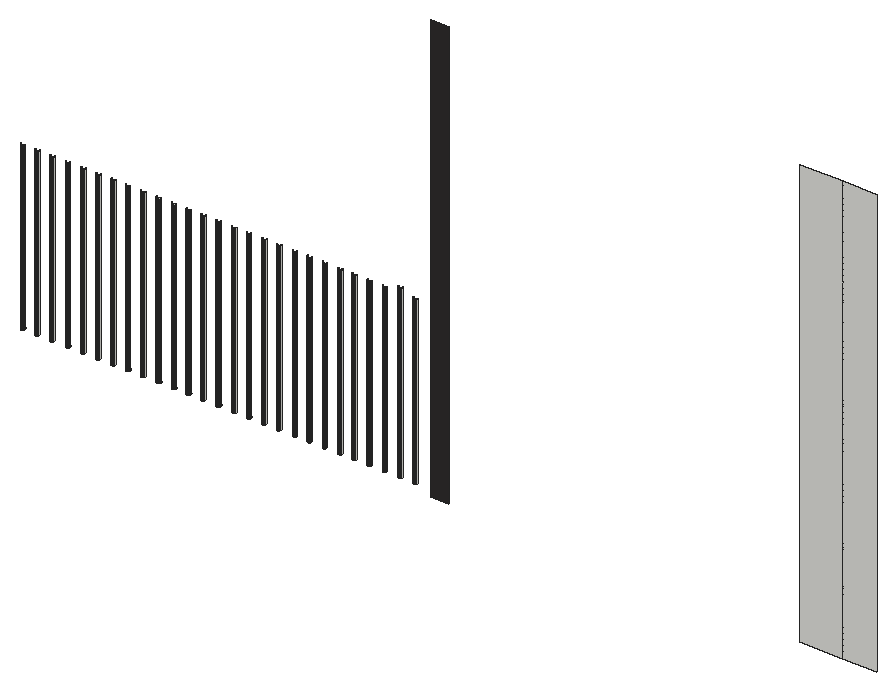
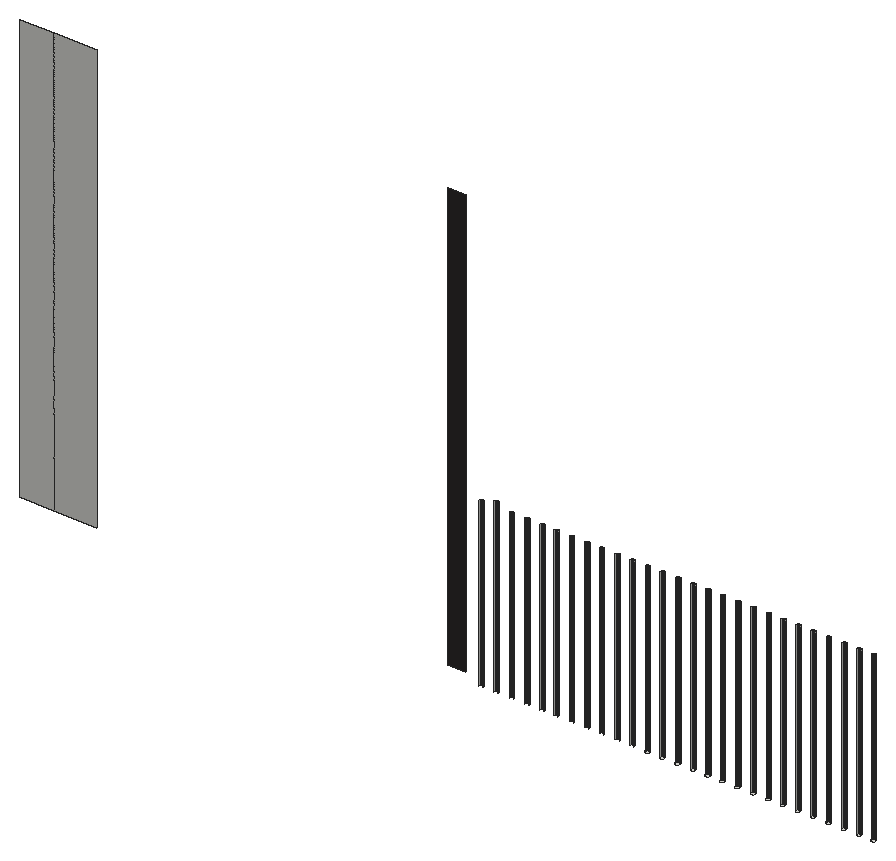
# SketchUp Ruby script. Lengths in inches.
U = 1.inch
M = Sketchup.active_model
def pt(a) = Geom::Point3d.new(a.map { |v| v * U })
def face(e, loops, mat)
  f = e.add_face(loops[0].map { |a| pt(a) })
  loops[1..].each { |l| e.add_face(l.map { |a| pt(a) }).erase! }
  f.material = f.back_material = mat if mat
  f
end
# faces: each face lists its corners as indices into pts; further lists are holes
def faces(e, pts, list, mat = nil) = list.each { |f| face(e, (f[0].is_a?(Array) ? f : [f]).map { |l| l.map { |i| pts[i] } }, mat) }
# xy, xz, yz: faces in a plane at the given z, y or x. An outline is a flat list of corners, or four numbers for a rectangle; further outlines are holes
def ring(l) = l.size == 4 ? [[l[0], l[1]], [l[2], l[1]], [l[2], l[3]], [l[0], l[3]]] : l.each_slice(2).to_a
def flat(e, list, mat, &to3) = list.each { |f| face(e, (f[0].is_a?(Array) ? f : [f]).map { |l| ring(l).map { |u, v| to3.(u, v) } }, mat) }
def xy(e, z, list, mat = nil) = flat(e, list, mat) { |x, y| [x, y, z] }
def xz(e, y, list, mat = nil) = flat(e, list, mat) { |x, z| [x, y, z] }
def yz(e, x, list, mat = nil) = flat(e, list, mat) { |y, z| [x, y, z] }
def lines(e, pts, list) = list.each { |a, b| e.add_line(pt(pts[a]), pt(pts[b])) }
# prism: a flat outline (further loops are holes) pulled along v
def prism(e, loops, v, mat = nil)
  f = face(e, loops, mat); d = Geom::Vector3d.new(v.map { |x| x * U })
  f.pushpull(f.normal.samedirection?(d) ? d.length : -d.length)
end
def box(e, o, s, mat = nil) = prism(e, [[o, [o[0] + s[0], o[1], o[2]], [o[0] + s[0], o[1] + s[1], o[2]], [o[0], o[1] + s[1], o[2]]]], [0, 0, s[2]], mat)
def at(x, y, z, deg = 0) = Geom::Transformation.translation(pt([x, y, z])) * Geom::Transformation.rotation(ORIGIN, Z_AXIS, deg.degrees)
def axes(o, x, y, z) = Geom::Transformation.new([*x, 0, *y, 0, *z, 0, *pt(o).to_a, 1])
def part(name) = M.definitions.add(name)
# library, detail: a bought-in or finely detailed component or shape, given as its bounding box
def library(name, o, s) = part(name).tap { |d| box(d.entities, o, s) }
def detail(e, o, s) = box(e.add_group.entities, o, s)
def put(e, d, t, mat = nil) = e.add_instance(d, t).tap { |i| i.material = mat if mat }
def group(e, t, mat = nil) = e.add_group.tap { |g| g.transformation = t; g.material = mat if mat }.entities
root = M.entities
M.materials.add("Generic\#4").color = [48, 45, 45]
xy(root,819.75,[[365.01,127.81,364.8,127.83,364.6,127.91,364.4375,128.04,364.31,128.21,364.23,128.41,364.2,128.62,364.23,128.83,364.31,129.02,364.4375,129.19,364.6,129.32,364.8,129.4,365.01,129.43,365.22,129.4,365.42,129.32,365.59,129.19,365.71,129.02,365.8,128.83,365.82,128.62,365.8,128.41,365.71,128.21,365.59,128.04,365.42,127.91,365.22,127.83],[370.76,127.81,370.55,127.83,370.35,127.91,370.1875,128.04,370.06,128.21,369.98,128.41,369.95,128.62,369.98,128.83,370.06,129.02,370.1875,129.19,370.35,129.32,370.55,129.4,370.76,129.43,370.97,129.4,371.17,129.32,371.34,129.19,371.46,129.02,371.55,128.83,371.57,128.62,371.55,128.41,371.46,128.21,371.34,128.04,371.17,127.91,370.97,127.83],[376.7,127.81,376.49,127.83,376.29,127.91,376.125,128.04,375.99,128.21,375.91,128.41,375.89,128.62,375.91,128.83,375.99,129.02,376.125,129.19,376.29,129.32,376.49,129.4,376.7,129.43,376.91,129.4,377.1,129.32,377.27,129.19,377.4,129.02,377.48,128.83,377.51,128.62,377.48,128.41,377.4,128.21,377.27,128.04,377.1,127.91,376.91,127.83],[382.76,127.81,382.55,127.83,382.35,127.91,382.1875,128.04,382.06,128.21,381.98,128.41,381.95,128.62,381.98,128.83,382.06,129.02,382.1875,129.19,382.35,129.32,382.55,129.4,382.76,129.43,382.97,129.4,383.17,129.32,383.34,129.19,383.46,129.02,383.55,128.83,383.57,128.62,383.55,128.41,383.46,128.21,383.34,128.04,383.17,127.91,382.97,127.83],[388.82,127.81,388.61,127.83,388.42,127.91,388.25,128.04,388.12,128.21,388.04,128.41,388.01,128.62,388.04,128.83,388.12,129.02,388.25,129.19,388.42,129.32,388.61,129.4,388.82,129.43,389.03,129.4,389.23,129.32,389.4,129.19,389.53,129.02,389.61,128.83,389.64,128.62,389.61,128.41,389.53,128.21,389.4,128.04,389.23,127.91,389.03,127.83],
  [394.76,127.81,394.55,127.83,394.35,127.91,394.1875,128.04,394.06,128.21,393.98,128.41,393.95,128.62,393.98,128.83,394.06,129.02,394.1875,129.19,394.35,129.32,394.55,129.4,394.76,129.43,394.97,129.4,395.17,129.32,395.34,129.19,395.46,129.02,395.55,128.83,395.57,128.62,395.55,128.41,395.46,128.21,395.34,128.04,395.17,127.91,394.97,127.83],[400.57,127.81,400.36,127.83,400.17,127.91,400,128.04,399.87,128.21,399.79,128.41,399.76,128.62,399.79,128.83,399.87,129.02,400,129.19,400.17,129.32,400.36,129.4,400.57,129.43,400.78,129.4,400.98,129.32,401.15,129.19,401.28,129.02,401.36,128.83,401.39,128.62,401.36,128.41,401.28,128.21,401.15,128.04,400.98,127.91,400.78,127.83],[406.39,127.81,406.18,127.83,405.98,127.91,405.8125,128.04,405.68,128.21,405.6,128.41,405.57,128.62,405.6,128.83,405.68,129.02,405.8125,129.19,405.98,129.32,406.18,129.4,406.39,129.43,406.6,129.4,406.79,129.32,406.96,129.19,407.09,129.02,407.17,128.83,407.2,128.62,407.17,128.41,407.09,128.21,406.96,128.04,406.79,127.91,406.6,127.83],[412.32,127.81,412.11,127.83,411.92,127.91,411.75,128.04,411.62,128.21,411.54,128.41,411.51,128.62,411.54,128.83,411.62,129.02,411.75,129.19,411.92,129.32,412.11,129.4,412.32,129.43,412.53,129.4,412.73,129.32,412.9,129.19,413.03,129.02,413.11,128.83,413.14,128.62,413.11,128.41,413.03,128.21,412.9,128.04,412.73,127.91,412.53,127.83],[418.45,127.81,418.24,127.83,418.04,127.91,417.875,128.04,417.74,128.21,417.66,128.41,417.64,128.62,417.66,128.83,417.74,129.02,417.875,129.19,418.04,129.32,418.24,129.4,418.45,129.43,418.66,129.4,418.85,129.32,419.02,129.19,419.15,129.02,419.23,128.83,419.26,128.62,419.23,128.41,419.15,128.21,419.02,128.04,418.85,127.91,418.66,127.83],
  [424.39,127.81,424.18,127.83,423.98,127.91,423.8125,128.04,423.68,128.21,423.6,128.41,423.57,128.62,423.6,128.83,423.68,129.02,423.8125,129.19,423.98,129.32,424.18,129.4,424.39,129.43,424.6,129.4,424.79,129.32,424.96,129.19,425.09,129.02,425.17,128.83,425.2,128.62,425.17,128.41,425.09,128.21,424.96,128.04,424.79,127.91,424.6,127.83],[430.2,127.81,429.99,127.83,429.79,127.91,429.625,128.04,429.49,128.21,429.41,128.41,429.39,128.62,429.41,128.83,429.49,129.02,429.625,129.19,429.79,129.32,429.99,129.4,430.2,129.43,430.41,129.4,430.6,129.32,430.77,129.19,430.9,129.02,430.98,128.83,431.01,128.62,430.98,128.41,430.9,128.21,430.77,128.04,430.6,127.91,430.41,127.83],[436.01,127.81,435.8,127.83,435.6,127.91,435.4375,128.04,435.31,128.21,435.23,128.41,435.2,128.62,435.23,128.83,435.31,129.02,435.4375,129.19,435.6,129.32,435.8,129.4,436.01,129.43,436.22,129.4,436.42,129.32,436.59,129.19,436.71,129.02,436.8,128.83,436.82,128.62,436.8,128.41,436.71,128.21,436.59,128.04,436.42,127.91,436.22,127.83],[442.01,127.81,441.8,127.83,441.6,127.91,441.4375,128.04,441.31,128.21,441.23,128.41,441.2,128.62,441.23,128.83,441.31,129.02,441.4375,129.19,441.6,129.32,441.8,129.4,442.01,129.43,442.22,129.4,442.42,129.32,442.59,129.19,442.71,129.02,442.8,128.83,442.82,128.62,442.8,128.41,442.71,128.21,442.59,128.04,442.42,127.91,442.22,127.83],[448.07,127.81,447.86,127.83,447.67,127.91,447.5,128.04,447.37,128.21,447.29,128.41,447.26,128.62,447.29,128.83,447.37,129.02,447.5,129.19,447.67,129.32,447.86,129.4,448.07,129.43,448.28,129.4,448.48,129.32,448.65,129.19,448.78,129.02,448.86,128.83,448.89,128.62,448.86,128.41,448.78,128.21,448.65,128.04,448.48,127.91,448.28,127.83],
  [453.89,127.81,453.68,127.83,453.48,127.91,453.3125,128.04,453.18,128.21,453.1,128.41,453.07,128.62,453.1,128.83,453.18,129.02,453.3125,129.19,453.48,129.32,453.68,129.4,453.89,129.43,454.1,129.4,454.29,129.32,454.46,129.19,454.59,129.02,454.67,128.83,454.7,128.62,454.67,128.41,454.59,128.21,454.46,128.04,454.29,127.91,454.1,127.83]])
xz(root,124.5,[[673.48,819.75,690.4375,987.75],[690.4375,819.75,703.6875,987.75]])
xz(root,124.5,[[528.75,819.75,535.75,987.75]],"Generic\#4")
p = [[364.6,127.91,819.75],[364.8,127.83,819.75],[364.8,127.83,884.89],[364.6,127.91,884.89],[365.01,127.81,819.75],[365.01,127.81,884.89],
  [365.22,127.83,819.75],[365.22,127.83,884.89],[365.42,127.91,819.75],[365.42,127.91,884.89],[370.35,127.91,819.75],[370.55,127.83,819.75],
  [370.55,127.83,884.89],[370.35,127.91,884.89],[370.76,127.81,819.75],[370.76,127.81,884.89],[370.97,127.83,819.75],[370.97,127.83,884.89],
  [371.17,127.91,819.75],[371.17,127.91,884.89],[376.29,127.91,819.75],[376.49,127.83,819.75],[376.49,127.83,884.89],[376.29,127.91,884.89],
  [376.7,127.81,819.75],[376.7,127.81,884.89],[376.91,127.83,819.75],[376.91,127.83,884.89],[377.1,127.91,819.75],[377.1,127.91,884.89],
  [382.35,127.91,819.75],[382.55,127.83,819.75],[382.55,127.83,884.89],[382.35,127.91,884.89],[382.76,127.81,819.75],[382.76,127.81,884.89],
  [382.97,127.83,819.75],[382.97,127.83,884.89],[383.17,127.91,819.75],[383.17,127.91,884.89],[388.42,127.91,819.75],[388.61,127.83,819.75],
  [388.61,127.83,884.89],[388.42,127.91,884.89],[388.82,127.81,819.75],[388.82,127.81,884.89],[389.03,127.83,819.75],[389.03,127.83,884.89],
  [389.23,127.91,819.75],[389.23,127.91,884.89],[394.35,127.91,819.75],[394.55,127.83,819.75],[394.55,127.83,884.89],[394.35,127.91,884.89],
  [394.76,127.81,819.75],[394.76,127.81,884.89],[394.97,127.83,819.75],[394.97,127.83,884.89],[395.17,127.91,819.75],[395.17,127.91,884.89],
  [400.17,127.91,819.75],[400.36,127.83,819.75],[400.36,127.83,884.89],[400.17,127.91,884.89],[400.57,127.81,819.75],[400.57,127.81,884.89],
  [400.78,127.83,819.75],[400.78,127.83,884.89],[400.98,127.91,819.75],[400.98,127.91,884.89],[405.98,127.91,819.75],[406.18,127.83,819.75],
  [406.18,127.83,884.89],[405.98,127.91,884.89],[406.39,127.81,819.75],[406.39,127.81,884.89],[406.6,127.83,819.75],[406.6,127.83,884.89],
  [406.79,127.91,819.75],[406.79,127.91,884.89],[411.92,127.91,819.75],[412.11,127.83,819.75],[412.11,127.83,884.89],[411.92,127.91,884.89],
  [412.32,127.81,819.75],[412.32,127.81,884.89],[412.53,127.83,819.75],[412.53,127.83,884.89],[412.73,127.91,819.75],[412.73,127.91,884.89],
  [418.04,127.91,819.75],[418.24,127.83,819.75],[418.24,127.83,884.89],[418.04,127.91,884.89],[418.45,127.81,819.75],[418.45,127.81,884.89],
  [418.66,127.83,819.75],[418.66,127.83,884.89],[418.85,127.91,819.75],[418.85,127.91,884.89],[423.98,127.91,819.75],[424.18,127.83,819.75],
  [424.18,127.83,884.89],[423.98,127.91,884.89],[424.39,127.81,819.75],[424.39,127.81,884.89],[424.6,127.83,819.75],[424.6,127.83,884.89],
  [424.79,127.91,819.75],[424.79,127.91,884.89],[429.79,127.91,819.75],[429.99,127.83,819.75],[429.99,127.83,884.89],[429.79,127.91,884.89],
  [430.2,127.81,819.75],[430.2,127.81,884.89],[430.41,127.83,819.75],[430.41,127.83,884.89],[430.6,127.91,819.75],[430.6,127.91,884.89],
  [435.6,127.91,819.75],[435.8,127.83,819.75],[435.8,127.83,884.89],[435.6,127.91,884.89],[436.01,127.81,819.75],[436.01,127.81,884.89],
  [436.22,127.83,819.75],[436.22,127.83,884.89],[436.42,127.91,819.75],[436.42,127.91,884.89],[441.6,127.91,819.75],[441.8,127.83,819.75],
  [441.8,127.83,884.89],[441.6,127.91,884.89],[442.01,127.81,819.75],[442.01,127.81,884.89],[442.22,127.83,819.75],[442.22,127.83,884.89],
  [442.42,127.91,819.75],[442.42,127.91,884.89],[447.67,127.91,819.75],[447.86,127.83,819.75],[447.86,127.83,884.89],[447.67,127.91,884.89],
  [448.07,127.81,819.75],[448.07,127.81,884.89],[448.28,127.83,819.75],[448.28,127.83,884.89],[448.48,127.91,819.75],[448.48,127.91,884.89],
  [453.48,127.91,819.75],[453.68,127.83,819.75],[453.68,127.83,884.89],[453.48,127.91,884.89],[453.89,127.81,819.75],[453.89,127.81,884.89],
  [454.1,127.83,819.75],[454.1,127.83,884.89],[454.29,127.91,819.75],[454.29,127.91,884.89],[459.54,127.91,819.75],[459.74,127.83,819.75],
  [459.74,127.83,884.89],[459.54,127.91,884.89],[459.95,127.81,819.75],[459.95,127.81,884.89],[460.16,127.83,819.75],[460.16,127.83,884.89],
  [460.35,127.91,819.75],[460.35,127.91,884.89],[465.35,127.91,819.75],[465.55,127.83,819.75],[465.55,127.83,884.89],[465.35,127.91,884.89],
  [465.76,127.81,819.75],[465.76,127.81,884.89],[465.97,127.83,819.75],[465.97,127.83,884.89],[466.17,127.91,819.75],[466.17,127.91,884.89],
  [471.54,127.91,819.75],[471.74,127.83,819.75],[471.74,127.83,884.89],[471.54,127.91,884.89],[471.95,127.81,819.75],[471.95,127.81,884.89],
  [472.16,127.83,819.75],[472.16,127.83,884.89],[472.35,127.91,819.75],[472.35,127.91,884.89],[477.35,127.91,819.75],[477.55,127.83,819.75],
  [477.55,127.83,884.89],[477.35,127.91,884.89],[477.76,127.81,819.75],[477.76,127.81,884.89],[477.97,127.83,819.75],[477.97,127.83,884.89],
  [478.17,127.91,819.75],[478.17,127.91,884.89],[483.35,127.91,819.75],[483.55,127.83,819.75],[483.55,127.83,884.89],[483.35,127.91,884.89],
  [483.76,127.81,819.75],[483.76,127.81,884.89],[483.97,127.83,819.75],[483.97,127.83,884.89],[484.17,127.91,819.75],[484.17,127.91,884.89],
  [489.48,127.91,819.75],[489.68,127.83,819.75],[489.68,127.83,884.89],[489.48,127.91,884.89],[489.89,127.81,819.75],[489.89,127.81,884.89],
  [490.1,127.83,819.75],[490.1,127.83,884.89],[490.29,127.91,819.75],[490.29,127.91,884.89],[494.98,127.91,819.75],[495.18,127.83,819.75],
  [495.18,127.83,884.89],[494.98,127.91,884.89],[495.39,127.81,819.75],[495.39,127.81,884.89],[495.6,127.83,819.75],[495.6,127.83,884.89],
  [495.79,127.91,819.75],[495.79,127.91,884.89],[500.92,127.91,819.75],[501.11,127.83,819.75],[501.11,127.83,884.89],[500.92,127.91,884.89],
  [501.32,127.81,819.75],[501.32,127.81,884.89],[501.53,127.83,819.75],[501.53,127.83,884.89],[501.73,127.91,819.75],[501.73,127.91,884.89],
  [506.98,127.91,819.75],[507.18,127.83,819.75],[507.18,127.83,884.89],[506.98,127.91,884.89],[507.39,127.81,819.75],[507.39,127.81,884.89],
  [507.6,127.83,819.75],[507.6,127.83,884.89],[507.79,127.91,819.75],[507.79,127.91,884.89],[513.04,127.91,819.75],[513.24,127.83,819.75],
  [513.24,127.83,886.75],[513.04,127.91,886.75],[513.45,127.81,819.75],[513.45,127.81,886.75],[513.66,127.83,819.75],[513.66,127.83,886.75],
  [513.85,127.91,819.75],[513.85,127.91,886.75],[518.92,127.91,819.75],[519.11,127.83,819.75],[519.11,127.83,884.89],[518.92,127.91,884.89],
  [519.32,127.81,819.75],[519.32,127.81,884.89],[519.53,127.83,819.75],[519.53,127.83,884.89],[519.73,127.91,819.75],[519.73,127.91,884.89],
  [364.4375,128.04,819.75],[364.4375,128.04,884.89],[365.59,128.04,819.75],[365.59,128.04,884.89],[370.1875,128.04,819.75],[370.1875,128.04,884.89],
  [371.34,128.04,819.75],[371.34,128.04,884.89],[376.125,128.04,819.75],[376.125,128.04,884.89],[377.27,128.04,819.75],[377.27,128.04,884.89],
  [382.1875,128.04,819.75],[382.1875,128.04,884.89],[383.34,128.04,819.75],[383.34,128.04,884.89],[388.25,128.04,819.75],[388.25,128.04,884.89],
  [389.4,128.04,819.75],[389.4,128.04,884.89],[394.1875,128.04,819.75],[394.1875,128.04,884.89],[395.34,128.04,819.75],[395.34,128.04,884.89],
  [400,128.04,819.75],[400,128.04,884.89],[401.15,128.04,819.75],[401.15,128.04,884.89],[405.8125,128.04,819.75],[405.8125,128.04,884.89],
  [406.96,128.04,819.75],[406.96,128.04,884.89],[411.75,128.04,819.75],[411.75,128.04,884.89],[412.9,128.04,819.75],[412.9,128.04,884.89],
  [417.875,128.04,819.75],[417.875,128.04,884.89],[419.02,128.04,819.75],[419.02,128.04,884.89],[423.8125,128.04,819.75],[423.8125,128.04,884.89],
  [424.96,128.04,819.75],[424.96,128.04,884.89],[429.625,128.04,819.75],[429.625,128.04,884.89],[430.77,128.04,819.75],[430.77,128.04,884.89],
  [435.4375,128.04,819.75],[435.4375,128.04,884.89],[436.59,128.04,819.75],[436.59,128.04,884.89],[441.4375,128.04,819.75],[441.4375,128.04,884.89],
  [442.59,128.04,819.75],[442.59,128.04,884.89],[447.5,128.04,819.75],[447.5,128.04,884.89],[448.65,128.04,819.75],[448.65,128.04,884.89],
  [453.3125,128.04,819.75],[453.3125,128.04,884.89],[454.46,128.04,819.75],[454.46,128.04,884.89],[459.375,128.04,819.75],[459.375,128.04,884.89],
  [460.52,128.04,819.75],[460.52,128.04,884.89],[465.1875,128.04,819.75],[465.1875,128.04,884.89],[466.34,128.04,819.75],[466.34,128.04,884.89],
  [471.375,128.04,819.75],[471.375,128.04,884.89],[472.52,128.04,819.75],[472.52,128.04,884.89],[477.1875,128.04,819.75],[477.1875,128.04,884.89],
  [478.34,128.04,819.75],[478.34,128.04,884.89],[483.1875,128.04,819.75],[483.1875,128.04,884.89],[484.34,128.04,819.75],[484.34,128.04,884.89],
  [489.3125,128.04,819.75],[489.3125,128.04,884.89],[490.46,128.04,819.75],[490.46,128.04,884.89],[494.8125,128.04,819.75],[494.8125,128.04,884.89],
  [495.96,128.04,819.75],[495.96,128.04,884.89],[500.75,128.04,819.75],[500.75,128.04,884.89],[501.9,128.04,819.75],[501.9,128.04,884.89],
  [506.8125,128.04,819.75],[506.8125,128.04,884.89],[507.96,128.04,819.75],[507.96,128.04,884.89],[512.875,128.04,819.75],[512.875,128.04,886.75],
  [514.02,128.04,819.75],[514.02,128.04,886.75],[518.75,128.04,819.75],[518.75,128.04,884.89],[519.9,128.04,819.75],[519.9,128.04,884.89],
  [364.31,128.21,819.75],[364.31,128.21,884.89],[365.71,128.21,819.75],[365.71,128.21,884.89],[370.06,128.21,819.75],[370.06,128.21,884.89],
  [371.46,128.21,819.75],[371.46,128.21,884.89],[375.99,128.21,819.75],[375.99,128.21,884.89],[377.4,128.21,819.75],[377.4,128.21,884.89],
  [382.06,128.21,819.75],[382.06,128.21,884.89],[383.46,128.21,819.75],[383.46,128.21,884.89],[388.12,128.21,819.75],[388.12,128.21,884.89],
  [389.53,128.21,819.75],[389.53,128.21,884.89],[394.06,128.21,819.75],[394.06,128.21,884.89],[395.46,128.21,819.75],[395.46,128.21,884.89],
  [399.87,128.21,819.75],[399.87,128.21,884.89],[401.28,128.21,819.75],[401.28,128.21,884.89],[405.68,128.21,819.75],[405.68,128.21,884.89],
  [407.09,128.21,819.75],[407.09,128.21,884.89],[411.62,128.21,819.75],[411.62,128.21,884.89],[413.03,128.21,819.75],[413.03,128.21,884.89],
  [417.74,128.21,819.75],[417.74,128.21,884.89],[419.15,128.21,819.75],[419.15,128.21,884.89],[423.68,128.21,819.75],[423.68,128.21,884.89],
  [425.09,128.21,819.75],[425.09,128.21,884.89],[429.49,128.21,819.75],[429.49,128.21,884.89],[430.9,128.21,819.75],[430.9,128.21,884.89],
  [435.31,128.21,819.75],[435.31,128.21,884.89],[436.71,128.21,819.75],[436.71,128.21,884.89],[441.31,128.21,819.75],[441.31,128.21,884.89],
  [442.71,128.21,819.75],[442.71,128.21,884.89],[447.37,128.21,819.75],[447.37,128.21,884.89],[448.78,128.21,819.75],[448.78,128.21,884.89],
  [453.18,128.21,819.75],[453.18,128.21,884.89],[454.59,128.21,819.75],[454.59,128.21,884.89],[459.24,128.21,819.75],[459.24,128.21,884.89],
  [460.65,128.21,819.75],[460.65,128.21,884.89],[465.06,128.21,819.75],[465.06,128.21,884.89],[466.46,128.21,819.75],[466.46,128.21,884.89],
  [471.24,128.21,819.75],[471.24,128.21,884.89],[472.65,128.21,819.75],[472.65,128.21,884.89],[477.06,128.21,819.75],[477.06,128.21,884.89],
  [478.46,128.21,819.75],[478.46,128.21,884.89],[483.06,128.21,819.75],[483.06,128.21,884.89],[484.46,128.21,819.75],[484.46,128.21,884.89],
  [489.18,128.21,819.75],[489.18,128.21,884.89],[490.59,128.21,819.75],[490.59,128.21,884.89],[494.68,128.21,819.75],[494.68,128.21,884.89],
  [496.09,128.21,819.75],[496.09,128.21,884.89],[500.62,128.21,819.75],[500.62,128.21,884.89],[502.03,128.21,819.75],[502.03,128.21,884.89],
  [506.68,128.21,819.75],[506.68,128.21,884.89],[508.09,128.21,819.75],[508.09,128.21,884.89],[512.74,128.21,819.75],[512.74,128.21,886.75],
  [514.15,128.21,819.75],[514.15,128.21,886.75],[518.62,128.21,819.75],[518.62,128.21,884.89],[520.03,128.21,819.75],[520.03,128.21,884.89],
  [364.23,128.41,819.75],[364.23,128.41,884.89],[365.8,128.41,819.75],[365.8,128.41,884.89],[369.98,128.41,819.75],[369.98,128.41,884.89],
  [371.55,128.41,819.75],[371.55,128.41,884.89],[375.91,128.41,819.75],[375.91,128.41,884.89],[377.48,128.41,819.75],[377.48,128.41,884.89],
  [381.98,128.41,819.75],[381.98,128.41,884.89],[383.55,128.41,819.75],[383.55,128.41,884.89],[388.04,128.41,819.75],[388.04,128.41,884.89],
  [389.61,128.41,819.75],[389.61,128.41,884.89],[393.98,128.41,819.75],[393.98,128.41,884.89],[395.55,128.41,819.75],[395.55,128.41,884.89],
  [399.79,128.41,819.75],[399.79,128.41,884.89],[401.36,128.41,819.75],[401.36,128.41,884.89],[405.6,128.41,819.75],[405.6,128.41,884.89],
  [407.17,128.41,819.75],[407.17,128.41,884.89],[411.54,128.41,819.75],[411.54,128.41,884.89],[413.11,128.41,819.75],[413.11,128.41,884.89],
  [417.66,128.41,819.75],[417.66,128.41,884.89],[419.23,128.41,819.75],[419.23,128.41,884.89],[423.6,128.41,819.75],[423.6,128.41,884.89],
  [425.17,128.41,819.75],[425.17,128.41,884.89],[429.41,128.41,819.75],[429.41,128.41,884.89],[430.98,128.41,819.75],[430.98,128.41,884.89],
  [435.23,128.41,819.75],[435.23,128.41,884.89],[436.8,128.41,819.75],[436.8,128.41,884.89],[441.23,128.41,819.75],[441.23,128.41,884.89],
  [442.8,128.41,819.75],[442.8,128.41,884.89],[447.29,128.41,819.75],[447.29,128.41,884.89],[448.86,128.41,819.75],[448.86,128.41,884.89],
  [453.1,128.41,819.75],[453.1,128.41,884.89],[454.67,128.41,819.75],[454.67,128.41,884.89],[459.16,128.41,819.75],[459.16,128.41,884.89],
  [460.73,128.41,819.75],[460.73,128.41,884.89],[464.98,128.41,819.75],[464.98,128.41,884.89],[466.55,128.41,819.75],[466.55,128.41,884.89],
  [471.16,128.41,819.75],[471.16,128.41,884.89],[472.73,128.41,819.75],[472.73,128.41,884.89],[476.98,128.41,819.75],[476.98,128.41,884.89],
  [478.55,128.41,819.75],[478.55,128.41,884.89],[482.98,128.41,819.75],[482.98,128.41,884.89],[484.55,128.41,819.75],[484.55,128.41,884.89],
  [489.1,128.41,819.75],[489.1,128.41,884.89],[490.67,128.41,819.75],[490.67,128.41,884.89],[494.6,128.41,819.75],[494.6,128.41,884.89],
  [496.17,128.41,819.75],[496.17,128.41,884.89],[500.54,128.41,819.75],[500.54,128.41,884.89],[502.11,128.41,819.75],[502.11,128.41,884.89],
  [506.6,128.41,819.75],[506.6,128.41,884.89],[508.17,128.41,819.75],[508.17,128.41,884.89],[512.66,128.41,819.75],[512.66,128.41,886.75],
  [514.23,128.41,819.75],[514.23,128.41,886.75],[518.54,128.41,819.75],[518.54,128.41,884.89],[520.11,128.41,819.75],[520.11,128.41,884.89],
  [364.2,128.62,819.75],[364.2,128.62,884.89],[365.82,128.62,819.75],[365.82,128.62,884.89],[369.95,128.62,819.75],[369.95,128.62,884.89],
  [371.57,128.62,819.75],[371.57,128.62,884.89],[375.89,128.62,819.75],[375.89,128.62,884.89],[377.51,128.62,819.75],[377.51,128.62,884.89],
  [381.95,128.62,819.75],[381.95,128.62,884.89],[383.57,128.62,819.75],[383.57,128.62,884.89],[388.01,128.62,819.75],[388.01,128.62,884.89],
  [389.64,128.62,819.75],[389.64,128.62,884.89],[393.95,128.62,819.75],[393.95,128.62,884.89],[395.57,128.62,819.75],[395.57,128.62,884.89],
  [399.76,128.62,819.75],[399.76,128.62,884.89],[401.39,128.62,819.75],[401.39,128.62,884.89],[405.57,128.62,819.75],[405.57,128.62,884.89],
  [407.2,128.62,819.75],[407.2,128.62,884.89],[411.51,128.62,819.75],[411.51,128.62,884.89],[413.14,128.62,819.75],[413.14,128.62,884.89],
  [417.64,128.62,819.75],[417.64,128.62,884.89],[419.26,128.62,819.75],[419.26,128.62,884.89],[423.57,128.62,819.75],[423.57,128.62,884.89],
  [425.2,128.62,819.75],[425.2,128.62,884.89],[429.39,128.62,819.75],[429.39,128.62,884.89],[431.01,128.62,819.75],[431.01,128.62,884.89],
  [435.2,128.62,819.75],[435.2,128.62,884.89],[436.82,128.62,819.75],[436.82,128.62,884.89],[441.2,128.62,819.75],[441.2,128.62,884.89],
  [442.82,128.62,819.75],[442.82,128.62,884.89],[447.26,128.62,819.75],[447.26,128.62,884.89],[448.89,128.62,819.75],[448.89,128.62,884.89],
  [453.07,128.62,819.75],[453.07,128.62,884.89],[454.7,128.62,819.75],[454.7,128.62,884.89],[459.14,128.62,819.75],[459.14,128.62,884.89],
  [460.76,128.62,819.75],[460.76,128.62,884.89],[464.95,128.62,819.75],[464.95,128.62,884.89],[466.57,128.62,819.75],[466.57,128.62,884.89],
  [471.14,128.62,819.75],[471.14,128.62,884.89],[472.76,128.62,819.75],[472.76,128.62,884.89],[476.95,128.62,819.75],[476.95,128.62,884.89],
  [478.57,128.62,819.75],[478.57,128.62,884.89],[482.95,128.62,819.75],[482.95,128.62,884.89],[484.57,128.62,819.75],[484.57,128.62,884.89],
  [489.07,128.62,819.75],[489.07,128.62,884.89],[490.7,128.62,819.75],[490.7,128.62,884.89],[494.57,128.62,819.75],[494.57,128.62,884.89],
  [496.2,128.62,819.75],[496.2,128.62,884.89],[500.51,128.62,819.75],[500.51,128.62,884.89],[502.14,128.62,819.75],[502.14,128.62,884.89],
  [506.57,128.62,819.75],[506.57,128.62,884.89],[508.2,128.62,819.75],[508.2,128.62,884.89],[512.64,128.62,819.75],[512.64,128.62,886.75],
  [514.26,128.62,819.75],[514.26,128.62,886.75],[518.51,128.62,819.75],[518.51,128.62,884.89],[520.14,128.62,819.75],[520.14,128.62,884.89]]
faces(root,p,[[0,1,2,3],[1,4,5,2],[4,6,7,5],[6,8,9,7],[10,11,12,13],[11,14,15,12],[14,16,17,15],[16,18,19,17],
  [20,21,22,23],[21,24,25,22],[24,26,27,25],[26,28,29,27],[30,31,32,33],[31,34,35,32],[34,36,37,35],[36,38,39,37],
  [40,41,42,43],[41,44,45,42],[44,46,47,45],[46,48,49,47],[50,51,52,53],[51,54,55,52],[54,56,57,55],[56,58,59,57],
  [60,61,62,63],[61,64,65,62],[64,66,67,65],[66,68,69,67],[70,71,72,73],[71,74,75,72],[74,76,77,75],[76,78,79,77],
  [80,81,82,83],[81,84,85,82],[84,86,87,85],[86,88,89,87],[90,91,92,93],[91,94,95,92],[94,96,97,95],[96,98,99,97],
  [100,101,102,103],[101,104,105,102],[104,106,107,105],[106,108,109,107],[110,111,112,113],[111,114,115,112],[114,116,117,115],[116,118,119,117],
  [120,121,122,123],[121,124,125,122],[124,126,127,125],[126,128,129,127],[130,131,132,133],[131,134,135,132],[134,136,137,135],[136,138,139,137],
  [140,141,142,143],[141,144,145,142],[144,146,147,145],[146,148,149,147],[150,151,152,153],[151,154,155,152],[154,156,157,155],[156,158,159,157],
  [160,161,162,163],[161,164,165,162],[164,166,167,165],[166,168,169,167],[170,171,172,173],[171,174,175,172],[174,176,177,175],[176,178,179,177],
  [180,181,182,183],[181,184,185,182],[184,186,187,185],[186,188,189,187],[190,191,192,193],[191,194,195,192],[194,196,197,195],[196,198,199,197],
  [200,201,202,203],[201,204,205,202],[204,206,207,205],[206,208,209,207],[210,211,212,213],[211,214,215,212],[214,216,217,215],[216,218,219,217],
  [220,221,222,223],[221,224,225,222],[224,226,227,225],[226,228,229,227],[230,231,232,233],[231,234,235,232],[234,236,237,235],[236,238,239,237],
  [240,241,242,243],[241,244,245,242],[244,246,247,245],[246,248,249,247],[250,251,252,253],[251,254,255,252],[254,256,257,255],[256,258,259,257],
  [260,261,262,263],[261,264,265,262],[264,266,267,265],[266,268,269,267],[270,0,3,271],[8,272,273,9],[274,10,13,275],[18,276,277,19],
  [278,20,23,279],[28,280,281,29],[282,30,33,283],[38,284,285,39],[286,40,43,287],[48,288,289,49],[290,50,53,291],[58,292,293,59],
  [294,60,63,295],[68,296,297,69],[298,70,73,299],[78,300,301,79],[302,80,83,303],[88,304,305,89],[306,90,93,307],[98,308,309,99],
  [310,100,103,311],[108,312,313,109],[314,110,113,315],[118,316,317,119],[318,120,123,319],[128,320,321,129],[322,130,133,323],[138,324,325,139],
  [326,140,143,327],[148,328,329,149],[330,150,153,331],[158,332,333,159],[334,160,163,335],[168,336,337,169],[338,170,173,339],[178,340,341,179],
  [342,180,183,343],[188,344,345,189],[346,190,193,347],[198,348,349,199],[350,200,203,351],[208,352,353,209],[354,210,213,355],[218,356,357,219],
  [358,220,223,359],[228,360,361,229],[362,230,233,363],[238,364,365,239],[366,240,243,367],[248,368,369,249],[370,250,253,371],[258,372,373,259],
  [374,260,263,375],[268,376,377,269],[378,270,271,379],[272,380,381,273],[382,274,275,383],[276,384,385,277],[386,278,279,387],[280,388,389,281],
  [390,282,283,391],[284,392,393,285],[394,286,287,395],[288,396,397,289],[398,290,291,399],[292,400,401,293],[402,294,295,403],[296,404,405,297],
  [406,298,299,407],[300,408,409,301],[410,302,303,411],[304,412,413,305],[414,306,307,415],[308,416,417,309],[418,310,311,419],[312,420,421,313],
  [422,314,315,423],[316,424,425,317],[426,318,319,427],[320,428,429,321],[430,322,323,431],[324,432,433,325],[434,326,327,435],[328,436,437,329],
  [438,330,331,439],[332,440,441,333],[442,334,335,443],[336,444,445,337],[446,338,339,447],[340,448,449,341],[450,342,343,451],[344,452,453,345],
  [454,346,347,455],[348,456,457,349],[458,350,351,459],[352,460,461,353],[462,354,355,463],[356,464,465,357],[466,358,359,467],[360,468,469,361],
  [470,362,363,471],[364,472,473,365],[474,366,367,475],[368,476,477,369],[478,370,371,479],[372,480,481,373],[482,374,375,483],[376,484,485,377],
  [486,378,379,487],[380,488,489,381],[490,382,383,491],[384,492,493,385],[494,386,387,495],[388,496,497,389],[498,390,391,499],[392,500,501,393],
  [502,394,395,503],[396,504,505,397],[506,398,399,507],[400,508,509,401],[510,402,403,511],[404,512,513,405],[514,406,407,515],[408,516,517,409],
  [518,410,411,519],[412,520,521,413],[522,414,415,523],[416,524,525,417],[526,418,419,527],[420,528,529,421],[530,422,423,531],[424,532,533,425],
  [534,426,427,535],[428,536,537,429],[538,430,431,539],[432,540,541,433],[542,434,435,543],[436,544,545,437],[546,438,439,547],[440,548,549,441],
  [550,442,443,551],[444,552,553,445],[554,446,447,555],[448,556,557,449],[558,450,451,559],[452,560,561,453],[562,454,455,563],[456,564,565,457],
  [566,458,459,567],[460,568,569,461],[570,462,463,571],[464,572,573,465],[574,466,467,575],[468,576,577,469],[578,470,471,579],[472,580,581,473],
  [582,474,475,583],[476,584,585,477],[586,478,479,587],[480,588,589,481],[590,482,483,591],[484,592,593,485],[594,486,487,595],[488,596,597,489],
  [598,490,491,599],[492,600,601,493],[602,494,495,603],[496,604,605,497],[606,498,499,607],[500,608,609,501],[610,502,503,611],[504,612,613,505],
  [614,506,507,615],[508,616,617,509],[618,510,511,619],[512,620,621,513],[622,514,515,623],[516,624,625,517],[626,518,519,627],[520,628,629,521],
  [630,522,523,631],[524,632,633,525],[634,526,527,635],[528,636,637,529],[638,530,531,639],[532,640,641,533],[642,534,535,643],[536,644,645,537],
  [646,538,539,647],[540,648,649,541],[650,542,543,651],[544,652,653,545],[654,546,547,655],[548,656,657,549],[658,550,551,659],[552,660,661,553],
  [662,554,555,663],[556,664,665,557],[666,558,559,667],[560,668,669,561],[670,562,563,671],[564,672,673,565],[674,566,567,675],[568,676,677,569],
  [678,570,571,679],[572,680,681,573],[682,574,575,683],[576,684,685,577],[686,578,579,687],[580,688,689,581],[690,582,583,691],[584,692,693,585],
  [694,586,587,695],[588,696,697,589],[698,590,591,699],[592,700,701,593]])
